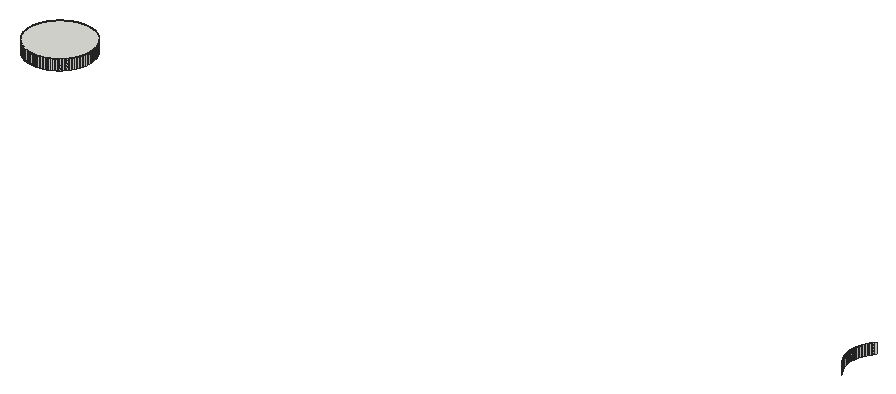
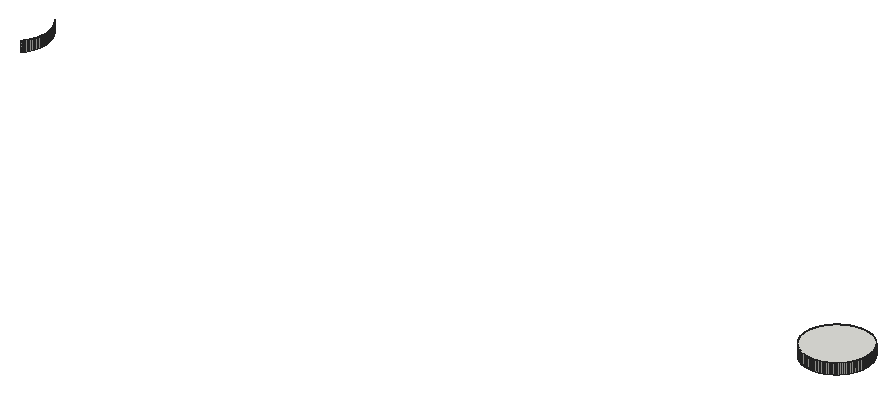
# SketchUp Ruby script. Lengths in inches.
U = 1.inch
M = Sketchup.active_model
def pt(a) = Geom::Point3d.new(a.map { |v| v * U })
def face(e, loops, mat)
  f = e.add_face(loops[0].map { |a| pt(a) })
  loops[1..].each { |l| e.add_face(l.map { |a| pt(a) }).erase! }
  f.material = f.back_material = mat if mat
  f
end
# faces: each face lists its corners as indices into pts; further lists are holes
def faces(e, pts, list, mat = nil) = list.each { |f| face(e, (f[0].is_a?(Array) ? f : [f]).map { |l| l.map { |i| pts[i] } }, mat) }
# xy, xz, yz: faces in a plane at the given z, y or x. An outline is a flat list of corners, or four numbers for a rectangle; further outlines are holes
def ring(l) = l.size == 4 ? [[l[0], l[1]], [l[2], l[1]], [l[2], l[3]], [l[0], l[3]]] : l.each_slice(2).to_a
def flat(e, list, mat, &to3) = list.each { |f| face(e, (f[0].is_a?(Array) ? f : [f]).map { |l| ring(l).map { |u, v| to3.(u, v) } }, mat) }
def xy(e, z, list, mat = nil) = flat(e, list, mat) { |x, y| [x, y, z] }
def xz(e, y, list, mat = nil) = flat(e, list, mat) { |x, z| [x, y, z] }
def yz(e, x, list, mat = nil) = flat(e, list, mat) { |y, z| [x, y, z] }
def lines(e, pts, list) = list.each { |a, b| e.add_line(pt(pts[a]), pt(pts[b])) }
# prism: a flat outline (further loops are holes) pulled along v
def prism(e, loops, v, mat = nil)
  f = face(e, loops, mat); d = Geom::Vector3d.new(v.map { |x| x * U })
  f.pushpull(f.normal.samedirection?(d) ? d.length : -d.length)
end
def box(e, o, s, mat = nil) = prism(e, [[o, [o[0] + s[0], o[1], o[2]], [o[0] + s[0], o[1] + s[1], o[2]], [o[0], o[1] + s[1], o[2]]]], [0, 0, s[2]], mat)
def at(x, y, z, deg = 0) = Geom::Transformation.translation(pt([x, y, z])) * Geom::Transformation.rotation(ORIGIN, Z_AXIS, deg.degrees)
def axes(o, x, y, z) = Geom::Transformation.new([*x, 0, *y, 0, *z, 0, *pt(o).to_a, 1])
def part(name) = M.definitions.add(name)
# library, detail: a bought-in or finely detailed component or shape, given as its bounding box
def library(name, o, s) = part(name).tap { |d| box(d.entities, o, s) }
def detail(e, o, s) = box(e.add_group.entities, o, s)
def put(e, d, t, mat = nil) = e.add_instance(d, t).tap { |i| i.material = mat if mat }
def group(e, t, mat = nil) = e.add_group.tap { |g| g.transformation = t; g.material = mat if mat }.entities
root = M.entities
xy(root,129,[[119.84,153,119.76,153.01,119.6875,153.02,119.61,153.03,119.45,153.05,119.375,153.07,119.3,153.08,119.22,153.1,119.15,153.125,119.07,153.15,119,153.17,118.92,153.2,118.71,153.29,118.64,153.33,118.57,153.36,118.43,153.44,118.37,153.48,118.3,153.53,118.24,153.57,118.17,153.62,117.93,153.82,117.88,153.88,117.82,153.93,117.62,154.17,117.57,154.24,117.53,154.3,117.48,154.37,117.44,154.43,117.36,154.57,117.33,154.64,117.29,154.71,117.2,154.92,117.17,155,117.15,155.07,117.125,155.15,117.1,155.22,117.08,155.3,117.07,155.375,117.05,155.45,117.03,155.61,117.02,155.6875,117.01,155.76,117,155.84,117,156.16,117.01,156.24,117.02,156.3125,117.03,156.39,117.05,156.55,117.07,156.625,117.08,156.7,117.1,156.78,117.125,156.85,117.15,156.93,117.17,157,117.2,157.08,117.29,157.29,117.33,157.36,117.36,157.43,117.44,157.57,117.48,157.63,117.53,157.7,117.57,157.76,117.62,157.83,117.82,158.07,117.88,158.12,117.93,158.18,118.17,158.38,118.24,158.43,118.3,158.47,118.37,158.52,118.43,158.56,118.57,158.64,118.64,158.67,118.71,158.71,118.92,158.8,119,158.83,119.07,158.85,119.15,158.875,119.22,158.9,119.3,158.92,119.375,158.93,119.45,158.95,119.61,158.97,119.6875,158.98,119.76,158.99,119.84,159,120.16,159,120.24,158.99,120.3125,158.98,120.39,158.97,120.55,158.95,120.625,158.93,120.7,158.92,120.78,158.9,120.85,158.875,120.93,158.85,121,158.83,121.08,158.8,121.29,158.71,121.36,158.67,121.43,158.64,121.57,158.56,121.63,158.52,121.7,158.47,121.76,158.43,121.83,158.38,122.07,158.18,122.12,158.12,122.18,158.07,122.38,157.83,122.43,157.76,122.47,157.7,122.52,157.63,122.56,157.57,122.64,157.43,122.67,157.36,122.71,157.29,122.8,157.08,122.83,157,122.85,156.93,122.875,156.85,122.9,156.78,122.92,156.7,122.93,156.625,122.95,156.55,122.97,156.39,122.98,156.3125,122.99,156.24,123,156.16,123,155.84,122.99,155.76,122.98,155.6875,122.97,155.61,122.95,155.45,122.93,155.375,122.92,155.3,122.9,155.22,122.875,155.15,122.85,155.07,122.83,155,122.8,154.92,122.71,154.71,122.67,154.64,122.64,154.57,122.56,154.43,122.52,154.37,122.47,154.3,122.43,154.24,122.38,154.17,122.18,153.93,122.12,153.88,122.07,153.82,121.83,153.62,121.76,153.57,121.7,153.53,121.63,153.48,121.57,153.44,121.43,153.36,121.36,153.33,121.29,153.29,121.08,153.2,121,153.17,120.93,153.15,120.85,153.125,120.78,153.1,120.7,153.08,120.625,153.07,120.55,153.05,120.39,153.03,120.3125,153.02,120.24,153.01,120.16,153]])
xz(root,153,[[119.84,128,119.92,129],[119.92,128,120,129],[120,128,120.08,129],[120.08,128,120.16,129]])
xz(root,159,[[119.84,128,119.92,129],[119.92,128,120,129],[120,128,120.08,129],[120.08,128,120.16,129]])
yz(root,117,[[155.84,128,155.92,129],[155.92,128,156,129],[156,128,156.08,129],[156.08,128,156.16,129]])
yz(root,123,[[155.84,128,155.92,129],[155.92,128,156,129],[156,128,156.08,129],[156.08,128,156.16,129]])
yz(root,197,[[155.84,128,155.92,129],[155.92,128,156,129],[156,128,156.08,129],[156.08,128,156.16,129]])
p = [[119.53,153.04,128],[119.45,153.05,128],[119.45,153.05,129],[119.53,153.04,129],[119.61,153.03,128],[119.61,153.03,129],
  [119.6875,153.02,128],[119.6875,153.02,129],[119.76,153.01,128],[119.76,153.01,129],[119.84,153,128],[119.84,153,129],
  [120.24,153.01,128],[120.16,153,128],[120.16,153,129],[120.24,153.01,129],[120.3125,153.02,128],[120.3125,153.02,129],
  [120.39,153.03,128],[120.39,153.03,129],[120.47,153.04,128],[120.47,153.04,129],[120.55,153.05,128],[120.55,153.05,129],
  [119.07,153.15,128],[119,153.17,128],[119,153.17,129],[119.07,153.15,129],[119.15,153.125,128],[119.15,153.125,129],
  [119.22,153.1,128],[119.22,153.1,129],[119.3,153.08,128],[119.3,153.08,129],[119.375,153.07,128],[119.375,153.07,129],
  [120.625,153.07,128],[120.625,153.07,129],[120.7,153.08,128],[120.7,153.08,129],[120.78,153.1,128],[120.78,153.1,129],
  [120.85,153.125,128],[120.85,153.125,129],[120.93,153.15,128],[120.93,153.15,129],[121,153.17,128],[121,153.17,129],
  [118.85,153.23,128],[118.78,153.26,128],[118.78,153.26,129],[118.85,153.23,129],[118.92,153.2,128],[118.92,153.2,129],
  [121.08,153.2,128],[121.08,153.2,129],[121.15,153.23,128],[121.15,153.23,129],[121.22,153.26,128],[121.22,153.26,129],
  [118.64,153.33,128],[118.57,153.36,128],[118.57,153.36,129],[118.64,153.33,129],[118.71,153.29,128],[118.71,153.29,129],
  [121.29,153.29,128],[121.29,153.29,129],[121.36,153.33,128],[121.36,153.33,129],[121.43,153.36,128],[121.43,153.36,129],
  [118.43,153.44,128],[118.37,153.48,128],[118.37,153.48,129],[118.43,153.44,129],[118.5,153.4,128],[118.5,153.4,129],
  [121.5,153.4,128],[121.5,153.4,129],[121.57,153.44,128],[121.57,153.44,129],[121.63,153.48,128],[121.63,153.48,129],
  [118.3,153.53,128],[118.24,153.57,128],[118.24,153.57,129],[118.3,153.53,129],[121.7,153.53,128],[121.7,153.53,129],
  [121.76,153.57,128],[121.76,153.57,129],[118.17,153.62,128],[118.11,153.67,128],[118.11,153.67,129],[118.17,153.62,129],
  [121.83,153.62,128],[121.83,153.62,129],[121.89,153.67,128],[121.89,153.67,129],[118.05,153.72,128],[117.99,153.77,128],
  [117.99,153.77,129],[118.05,153.72,129],[121.95,153.72,128],[121.95,153.72,129],[122.01,153.77,128],[122.01,153.77,129],
  [117.93,153.82,128],[117.88,153.88,128],[117.88,153.88,129],[117.93,153.82,129],[122.07,153.82,128],[122.07,153.82,129],
  [122.12,153.88,128],[122.12,153.88,129],[117.82,153.93,128],[117.77,153.99,128],[117.77,153.99,129],[117.82,153.93,129],
  [122.18,153.93,128],[122.18,153.93,129],[122.23,153.99,128],[122.23,153.99,129],[117.72,154.05,128],[117.72,154.05,129],
  [122.28,154.05,128],[122.28,154.05,129],[197.77,153.99,128],[197.72,154.05,128],[197.72,154.05,129],[197.77,153.99,129],
  [117.67,154.11,128],[117.62,154.17,128],[117.62,154.17,129],[117.67,154.11,129],[122.33,154.11,128],[122.33,154.11,129],
  [122.38,154.17,128],[122.38,154.17,129],[197.67,154.11,128],[197.62,154.17,128],[197.62,154.17,129],[197.67,154.11,129],
  [117.57,154.24,128],[117.53,154.3,128],[117.53,154.3,129],[117.57,154.24,129],[122.43,154.24,128],[122.43,154.24,129],
  [122.47,154.3,128],[122.47,154.3,129],[197.57,154.24,128],[197.53,154.3,128],[197.53,154.3,129],[197.57,154.24,129],
  [117.48,154.37,128],[117.48,154.37,129],[122.52,154.37,128],[122.52,154.37,129],[197.48,154.37,128],[197.48,154.37,129],
  [117.44,154.43,128],[117.4,154.5,128],[117.4,154.5,129],[117.44,154.43,129],[122.56,154.43,128],[122.56,154.43,129],
  [122.6,154.5,128],[122.6,154.5,129],[197.44,154.43,128],[197.4,154.5,128],[197.4,154.5,129],[197.44,154.43,129],
  [117.36,154.57,128],[117.36,154.57,129],[122.64,154.57,128],[122.64,154.57,129],[197.36,154.57,128],[197.36,154.57,129],
  [117.33,154.64,128],[117.29,154.71,128],[117.29,154.71,129],[117.33,154.64,129],[122.67,154.64,128],[122.67,154.64,129],
  [122.71,154.71,128],[122.71,154.71,129],[197.33,154.64,128],[197.29,154.71,128],[197.29,154.71,129],[197.33,154.64,129],
  [117.26,154.78,128],[117.26,154.78,129],[122.74,154.78,128],[122.74,154.78,129],[197.26,154.78,128],[197.26,154.78,129],
  [117.23,154.85,128],[117.23,154.85,129],[122.77,154.85,128],[122.77,154.85,129],[197.23,154.85,128],[197.23,154.85,129],
  [117.2,154.92,128],[117.17,155,128],[117.17,155,129],[117.2,154.92,129],[122.8,154.92,128],[122.8,154.92,129],
  [122.83,155,128],[122.83,155,129],[197.2,154.92,128],[197.17,155,128],[197.17,155,129],[197.2,154.92,129],
  [117.15,155.07,128],[117.15,155.07,129],[122.85,155.07,128],[122.85,155.07,129],[197.15,155.07,128],[197.15,155.07,129],
  [117.125,155.15,128],[117.1,155.22,128],[117.1,155.22,129],[117.125,155.15,129],[122.875,155.15,128],[122.875,155.15,129],
  [122.9,155.22,128],[122.9,155.22,129],[197.125,155.15,128],[197.1,155.22,128],[197.1,155.22,129],[197.125,155.15,129],
  [117.08,155.3,128],[117.08,155.3,129],[122.92,155.3,128],[122.92,155.3,129],[197.08,155.3,128],[197.08,155.3,129],
  [117.07,155.375,128],[117.07,155.375,129],[122.93,155.375,128],[122.93,155.375,129],[197.07,155.375,128],[197.07,155.375,129],
  [117.05,155.45,128],[117.05,155.45,129],[122.95,155.45,128],[122.95,155.45,129],[197.05,155.45,128],[197.05,155.45,129],
  [117.04,155.53,128],[117.03,155.61,128],[117.03,155.61,129],[117.04,155.53,129],[122.96,155.53,128],[122.96,155.53,129],
  [122.97,155.61,128],[122.97,155.61,129],[197.04,155.53,128],[197.03,155.61,128],[197.03,155.61,129],[197.04,155.53,129],
  [117.02,155.6875,128],[117.02,155.6875,129],[122.98,155.6875,128],[122.98,155.6875,129],[197.02,155.6875,128],[197.02,155.6875,129],
  [117.01,155.76,128],[117.01,155.76,129],[122.99,155.76,128],[122.99,155.76,129],[197.01,155.76,128],[197.01,155.76,129],
  [117,155.84,128],[117,155.84,129],[123,155.84,128],[123,155.84,129],[197,155.84,128],[197,155.84,129],
  [117,156.16,128],[117.01,156.24,128],[117.01,156.24,129],[117,156.16,129],[117.02,156.3125,128],[117.02,156.3125,129],
  [122.98,156.3125,128],[122.99,156.24,128],[122.99,156.24,129],[122.98,156.3125,129],[123,156.16,128],[123,156.16,129],
  [197,156.16,128],[197.01,156.24,128],[197.01,156.24,129],[197,156.16,129],[197.02,156.3125,128],[197.02,156.3125,129],
  [117.03,156.39,128],[117.03,156.39,129],[122.97,156.39,128],[122.97,156.39,129],[197.03,156.39,128],[197.03,156.39,129],
  [117.04,156.47,128],[117.04,156.47,129],[122.96,156.47,128],[122.96,156.47,129],[197.04,156.47,128],[197.04,156.47,129],
  [117.05,156.55,128],[117.05,156.55,129],[117.07,156.625,128],[117.07,156.625,129],[122.93,156.625,128],[122.95,156.55,128],
  [122.95,156.55,129],[122.93,156.625,129],[197.05,156.55,128],[197.05,156.55,129],[197.07,156.625,128],[197.07,156.625,129],
  [117.08,156.7,128],[117.08,156.7,129],[122.92,156.7,128],[122.92,156.7,129],[197.08,156.7,128],[197.08,156.7,129],
  [117.1,156.78,128],[117.1,156.78,129],[122.9,156.78,128],[122.9,156.78,129],[197.1,156.78,128],[197.1,156.78,129],
  [117.125,156.85,128],[117.125,156.85,129],[122.875,156.85,128],[122.875,156.85,129],[197.125,156.85,128],[197.125,156.85,129],
  [117.15,156.93,128],[117.15,156.93,129],[117.17,157,128],[117.17,157,129],[122.83,157,128],[122.85,156.93,128],
  [122.85,156.93,129],[122.83,157,129],[197.15,156.93,128],[197.15,156.93,129],[197.17,157,128],[197.17,157,129],
  [117.2,157.08,128],[117.2,157.08,129],[122.8,157.08,128],[122.8,157.08,129],[197.2,157.08,128],[197.2,157.08,129],
  [117.23,157.15,128],[117.23,157.15,129],[117.26,157.22,128],[117.26,157.22,129],[122.74,157.22,128],[122.77,157.15,128],
  [122.77,157.15,129],[122.74,157.22,129],[197.23,157.15,128],[197.23,157.15,129],[197.26,157.22,128],[197.26,157.22,129],
  [117.29,157.29,128],[117.29,157.29,129],[122.71,157.29,128],[122.71,157.29,129],[197.29,157.29,128],[197.29,157.29,129],
  [117.33,157.36,128],[117.33,157.36,129],[122.67,157.36,128],[122.67,157.36,129],[197.33,157.36,128],[197.33,157.36,129],
  [117.36,157.43,128],[117.36,157.43,129],[117.4,157.5,128],[117.4,157.5,129],[122.6,157.5,128],[122.64,157.43,128],
  [122.64,157.43,129],[122.6,157.5,129],[197.36,157.43,128],[197.36,157.43,129],[197.4,157.5,128],[197.4,157.5,129],
  [117.44,157.57,128],[117.44,157.57,129],[122.56,157.57,128],[122.56,157.57,129],[197.44,157.57,128],[197.44,157.57,129],
  [117.48,157.63,128],[117.48,157.63,129],[117.53,157.7,128],[117.53,157.7,129],[122.47,157.7,128],[122.52,157.63,128],
  [122.52,157.63,129],[122.47,157.7,129],[197.48,157.63,128],[197.48,157.63,129],[197.53,157.7,128],[197.53,157.7,129],
  [117.57,157.76,128],[117.57,157.76,129],[122.43,157.76,128],[122.43,157.76,129],[197.57,157.76,128],[197.57,157.76,129],
  [117.62,157.83,128],[117.62,157.83,129],[117.67,157.89,128],[117.67,157.89,129],[122.33,157.89,128],[122.38,157.83,128],
  [122.38,157.83,129],[122.33,157.89,129],[197.62,157.83,128],[197.62,157.83,129],[197.67,157.89,128],[197.67,157.89,129],
  [117.72,157.95,128],[117.72,157.95,129],[117.77,158.01,128],[117.77,158.01,129],[122.23,158.01,128],[122.28,157.95,128],
  [122.28,157.95,129],[122.23,158.01,129],[197.72,157.95,128],[197.72,157.95,129],[197.77,158.01,128],[197.77,158.01,129],
  [117.82,158.07,128],[117.82,158.07,129],[122.18,158.07,128],[122.18,158.07,129],[197.82,158.07,128],[197.82,158.07,129],
  [117.88,158.12,128],[117.88,158.12,129],[117.93,158.18,128],[117.93,158.18,129],[122.07,158.18,128],[122.12,158.12,128],
  [122.12,158.12,129],[122.07,158.18,129],[117.99,158.23,128],[117.99,158.23,129],[118.05,158.28,128],[118.05,158.28,129],
  [121.95,158.28,128],[122.01,158.23,128],[122.01,158.23,129],[121.95,158.28,129],[118.11,158.33,128],[118.11,158.33,129],
  [118.17,158.38,128],[118.17,158.38,129],[121.83,158.38,128],[121.89,158.33,128],[121.89,158.33,129],[121.83,158.38,129],
  [118.24,158.43,128],[118.24,158.43,129],[118.3,158.47,128],[118.3,158.47,129],[121.7,158.47,128],[121.76,158.43,128],
  [121.76,158.43,129],[121.7,158.47,129],[118.37,158.52,128],[118.37,158.52,129],[118.43,158.56,128],[118.43,158.56,129],
  [121.57,158.56,128],[121.63,158.52,128],[121.63,158.52,129],[121.57,158.56,129],[118.5,158.6,128],[118.5,158.6,129],
  [118.57,158.64,128],[118.57,158.64,129],[118.64,158.67,128],[118.64,158.67,129],[121.36,158.67,128],[121.43,158.64,128],
  [121.43,158.64,129],[121.36,158.67,129],[121.5,158.6,128],[121.5,158.6,129],[118.71,158.71,128],[118.71,158.71,129],
  [118.78,158.74,128],[118.78,158.74,129],[118.85,158.77,128],[118.85,158.77,129],[121.15,158.77,128],[121.22,158.74,128],
  [121.22,158.74,129],[121.15,158.77,129],[121.29,158.71,128],[121.29,158.71,129],[118.92,158.8,128],[118.92,158.8,129],
  [119,158.83,128],[119,158.83,129],[119.07,158.85,128],[119.07,158.85,129],[120.93,158.85,128],[121,158.83,128],
  [121,158.83,129],[120.93,158.85,129],[121.08,158.8,128],[121.08,158.8,129],[119.15,158.875,128],[119.15,158.875,129],
  [119.22,158.9,128],[119.22,158.9,129],[119.3,158.92,128],[119.3,158.92,129],[119.375,158.93,128],[119.375,158.93,129],
  [119.45,158.95,128],[119.45,158.95,129],[119.53,158.96,128],[119.53,158.96,129],[120.47,158.96,128],[120.55,158.95,128],
  [120.55,158.95,129],[120.47,158.96,129],[120.625,158.93,128],[120.625,158.93,129],[120.7,158.92,128],[120.7,158.92,129],
  [120.78,158.9,128],[120.78,158.9,129],[120.85,158.875,128],[120.85,158.875,129],[119.61,158.97,128],[119.61,158.97,129],
  [119.6875,158.98,128],[119.6875,158.98,129],[119.76,158.99,128],[119.76,158.99,129],[119.84,159,128],[119.84,159,129],
  [120.16,159,128],[120.24,158.99,128],[120.24,158.99,129],[120.16,159,129],[120.3125,158.98,128],[120.3125,158.98,129],
  [120.39,158.97,128],[120.39,158.97,129]]
faces(root,p,[[0,1,2,3],[4,0,3,5],[6,4,5,7],[8,6,7,9],[10,8,9,11],[12,13,14,15],[16,12,15,17],[18,16,17,19],
  [20,18,19,21],[22,20,21,23],[24,25,26,27],[28,24,27,29],[30,28,29,31],[32,30,31,33],[34,32,33,35],[1,34,35,2],
  [36,22,23,37],[38,36,37,39],[40,38,39,41],[42,40,41,43],[44,42,43,45],[46,44,45,47],[48,49,50,51],[52,48,51,53],
  [25,52,53,26],[54,46,47,55],[56,54,55,57],[58,56,57,59],[60,61,62,63],[64,60,63,65],[49,64,65,50],[66,58,59,67],
  [68,66,67,69],[70,68,69,71],[72,73,74,75],[76,72,75,77],[61,76,77,62],[78,70,71,79],[80,78,79,81],[82,80,81,83],
  [84,85,86,87],[73,84,87,74],[88,82,83,89],[90,88,89,91],[92,93,94,95],[85,92,95,86],[96,90,91,97],[98,96,97,99],
  [100,101,102,103],[93,100,103,94],[104,98,99,105],[106,104,105,107],[108,109,110,111],[101,108,111,102],[112,106,107,113],[114,112,113,115],
  [116,117,118,119],[109,116,119,110],[120,114,115,121],[122,120,121,123],[117,124,125,118],[126,122,123,127],[128,129,130,131],[132,133,134,135],
  [124,132,135,125],[136,126,127,137],[138,136,137,139],[140,141,142,143],[129,140,143,130],[144,145,146,147],[133,144,147,134],[148,138,139,149],
  [150,148,149,151],[152,153,154,155],[141,152,155,142],[145,156,157,146],[158,150,151,159],[153,160,161,154],[162,163,164,165],[156,162,165,157],
  [166,158,159,167],[168,166,167,169],[170,171,172,173],[160,170,173,161],[163,174,175,164],[176,168,169,177],[171,178,179,172],[180,181,182,183],
  [174,180,183,175],[184,176,177,185],[186,184,185,187],[188,189,190,191],[178,188,191,179],[181,192,193,182],[194,186,187,195],[189,196,197,190],
  [192,198,199,193],[200,194,195,201],[196,202,203,197],[204,205,206,207],[198,204,207,199],[208,200,201,209],[210,208,209,211],[212,213,214,215],
  [202,212,215,203],[205,216,217,206],[218,210,211,219],[213,220,221,214],[222,223,224,225],[216,222,225,217],[226,218,219,227],[228,226,227,229],
  [230,231,232,233],[220,230,233,221],[223,234,235,224],[236,228,229,237],[231,238,239,232],[234,240,241,235],[242,236,237,243],[238,244,245,239],
  [240,246,247,241],[248,242,243,249],[244,250,251,245],[252,253,254,255],[246,252,255,247],[256,248,249,257],[258,256,257,259],[260,261,262,263],
  [250,260,263,251],[253,264,265,254],[266,258,259,267],[261,268,269,262],[264,270,271,265],[272,266,267,273],[268,274,275,269],[270,276,277,271],
  [278,272,273,279],[274,280,281,275],[282,283,284,285],[283,286,287,284],[288,289,290,291],[289,292,293,290],[294,295,296,297],[295,298,299,296],
  [286,300,301,287],[302,288,291,303],[298,304,305,299],[300,306,307,301],[308,302,303,309],[304,310,311,305],[306,312,313,307],[312,314,315,313],
  [316,317,318,319],[317,308,309,318],[310,320,321,311],[320,322,323,321],[314,324,325,315],[326,316,319,327],[322,328,329,323],[324,330,331,325],
  [332,326,327,333],[328,334,335,329],[330,336,337,331],[338,332,333,339],[334,340,341,335],[336,342,343,337],[342,344,345,343],[346,347,348,349],
  [347,338,339,348],[340,350,351,341],[350,352,353,351],[344,354,355,345],[356,346,349,357],[352,358,359,353],[354,360,361,355],[360,362,363,361],
  [364,365,366,367],[365,356,357,366],[358,368,369,359],[368,370,371,369],[362,372,373,363],[374,364,367,375],[370,376,377,371],[372,378,379,373],
  [380,374,375,381],[376,382,383,377],[378,384,385,379],[384,386,387,385],[388,389,390,391],[389,380,381,390],[382,392,393,383],[392,394,395,393],
  [386,396,397,387],[398,388,391,399],[394,400,401,395],[396,402,403,397],[402,404,405,403],[406,407,408,409],[407,398,399,408],[400,410,411,401],
  [410,412,413,411],[404,414,415,405],[416,406,409,417],[412,418,419,413],[414,420,421,415],[420,422,423,421],[424,425,426,427],[425,416,417,426],
  [418,428,429,419],[428,430,431,429],[422,432,433,423],[432,434,435,433],[436,437,438,439],[437,424,427,438],[430,440,441,431],[440,442,443,441],
  [434,444,445,435],[446,436,439,447],[442,448,449,443],[444,450,451,445],[450,452,453,451],[454,455,456,457],[455,446,447,456],[452,458,459,453],
  [458,460,461,459],[462,463,464,465],[463,454,457,464],[460,466,467,461],[466,468,469,467],[470,471,472,473],[471,462,465,472],[468,474,475,469],
  [474,476,477,475],[478,479,480,481],[479,470,473,480],[476,482,483,477],[482,484,485,483],[486,487,488,489],[487,478,481,488],[484,490,491,485],
  [490,492,493,491],[492,494,495,493],[496,497,498,499],[497,500,501,498],[500,486,489,501],[494,502,503,495],[502,504,505,503],[504,506,507,505],
  [508,509,510,511],[509,512,513,510],[512,496,499,513],[506,514,515,507],[514,516,517,515],[516,518,519,517],[520,521,522,523],[521,524,525,522],
  [524,508,511,525],[518,526,527,519],[526,528,529,527],[528,530,531,529],[530,532,533,531],[532,534,535,533],[534,536,537,535],[538,539,540,541],
  [539,542,543,540],[542,544,545,543],[544,546,547,545],[546,548,549,547],[548,520,523,549],[536,550,551,537],[550,552,553,551],[552,554,555,553],
  [554,556,557,555],[558,559,560,561],[559,562,563,560],[562,564,565,563],[564,538,541,565]])
